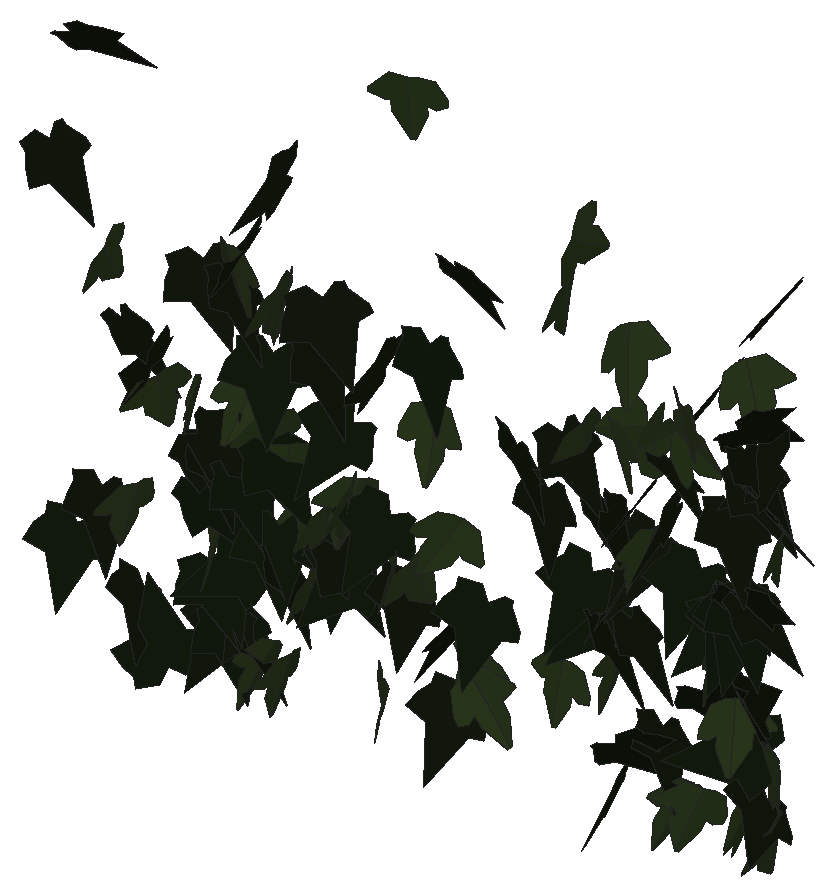
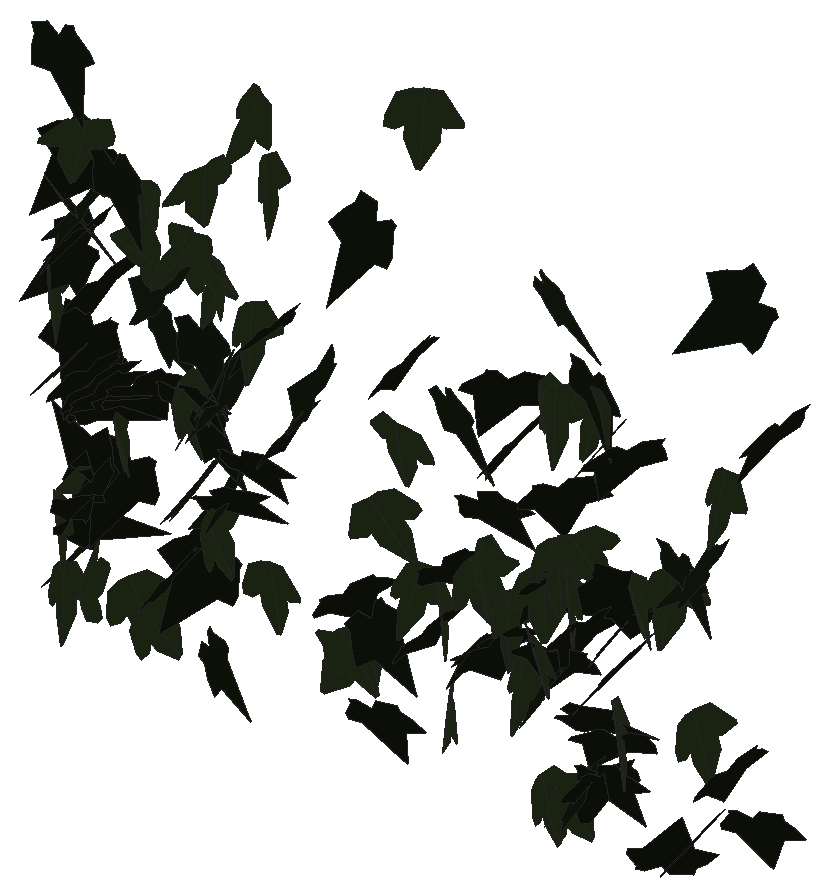
# SketchUp Ruby script. Lengths in inches.
U = 1.inch
M = Sketchup.active_model
def pt(a) = Geom::Point3d.new(a.map { |v| v * U })
def face(e, loops, mat)
  f = e.add_face(loops[0].map { |a| pt(a) })
  loops[1..].each { |l| e.add_face(l.map { |a| pt(a) }).erase! }
  f.material = f.back_material = mat if mat
  f
end
# faces: each face lists its corners as indices into pts; further lists are holes
def faces(e, pts, list, mat = nil) = list.each { |f| face(e, (f[0].is_a?(Array) ? f : [f]).map { |l| l.map { |i| pts[i] } }, mat) }
# xy, xz, yz: faces in a plane at the given z, y or x. An outline is a flat list of corners, or four numbers for a rectangle; further outlines are holes
def ring(l) = l.size == 4 ? [[l[0], l[1]], [l[2], l[1]], [l[2], l[3]], [l[0], l[3]]] : l.each_slice(2).to_a
def flat(e, list, mat, &to3) = list.each { |f| face(e, (f[0].is_a?(Array) ? f : [f]).map { |l| ring(l).map { |u, v| to3.(u, v) } }, mat) }
def xy(e, z, list, mat = nil) = flat(e, list, mat) { |x, y| [x, y, z] }
def xz(e, y, list, mat = nil) = flat(e, list, mat) { |x, z| [x, y, z] }
def yz(e, x, list, mat = nil) = flat(e, list, mat) { |y, z| [x, y, z] }
def lines(e, pts, list) = list.each { |a, b| e.add_line(pt(pts[a]), pt(pts[b])) }
# prism: a flat outline (further loops are holes) pulled along v
def prism(e, loops, v, mat = nil)
  f = face(e, loops, mat); d = Geom::Vector3d.new(v.map { |x| x * U })
  f.pushpull(f.normal.samedirection?(d) ? d.length : -d.length)
end
def box(e, o, s, mat = nil) = prism(e, [[o, [o[0] + s[0], o[1], o[2]], [o[0] + s[0], o[1] + s[1], o[2]], [o[0], o[1] + s[1], o[2]]]], [0, 0, s[2]], mat)
def at(x, y, z, deg = 0) = Geom::Transformation.translation(pt([x, y, z])) * Geom::Transformation.rotation(ORIGIN, Z_AXIS, deg.degrees)
def axes(o, x, y, z) = Geom::Transformation.new([*x, 0, *y, 0, *z, 0, *pt(o).to_a, 1])
def part(name) = M.definitions.add(name)
# library, detail: a bought-in or finely detailed component or shape, given as its bounding box
def library(name, o, s) = part(name).tap { |d| box(d.entities, o, s) }
def detail(e, o, s) = box(e.add_group.entities, o, s)
def put(e, d, t, mat = nil) = e.add_instance(d, t).tap { |i| i.material = mat if mat }
def group(e, t, mat = nil) = e.add_group.tap { |g| g.transformation = t; g.material = mat if mat }.entities
root = M.entities
M.materials.add("efeu1").color = [18, 25, 13]
M.materials.add("efeu2").color = [43, 57, 29]
c1 = part("ivyleaf_9")
p = [[1.54,2.16,1.25],[1.36,2.04,1.19],[-0.21,0.99,0.68],[-0.71,1.11,0.82],[-0.85,0.86,0.67],[-0.8,0.17,0.21],
  [-0.9,-0.01,0.1],[-0.67,-0.16,-0.02],[-0.08,-0.08,-0.05],[-0.03,-0.6,-0.4],[0.65,-0.88,-0.66],[0.83,-0.6,-0.49],
  [1.29,-0.42,-0.43],[1.8125,-0.07,-0.26],[1.21,0.44,0.15]]
faces(c1.entities,p,[[0,1,2,3,4,5,6,7,8,9,10,11,12,13,14]],"efeu1")
c2 = part("ivyleaf_10")
p = [[0,0.5,-0.03],[-0.0625,2.02,-0.43],[-0.19,2.01,-0.46],[-0.54,1.05,-0.29],[-0.52,0.625,-0.18],[-0.83,0.76,-0.28],
  [-1.16,0.64,-0.33],[-1.15,0.33,-0.24],[-0.77,-0.39,0.02],[-0.3,-0.51,0.16],[0.04,-0.48,0.23],[-0.02,2.01,-0.4375],
  [-0.06,2.01,-0.43],[0.04,-0.49,0.23],[0.67,-0.49,0.14],[1.38,0.36,-0.2],[1.375,0.51,-0.24],[0.81,0.65,-0.19],
  [0.62,0.59,-0.15],[0.6,1.09,-0.28],[0.5,1.23,-0.31]]
faces(c2.entities,p,[[0,1,2,3,4,5,6,7,8,9,10],[11,12,0,13,14,15,16,17,18,19,20]],"efeu2")
put(root,c1,axes([570.51,128.33,246.2],[0.79175,0.67685,0.12793],[0.09938,0.08063,-1.04162],[-0.68162,0.79795,-0.00327]))
put(root,c1,axes([574.61,129.34,255.92],[0.09837,-1.07427,-0.09221],[-0.0039,0.09224,-1.07876],[1.07822,0.09834,0.00451]))
put(root,c2,axes([560.36,128.3,244.3125],[0.17872,-0.33915,-0.98707],[-0.29964,0.94261,-0.37813],[0.99977,0.34313,0.06312]))
put(root,c2,axes([555.7,129.05,258.01],[0.38953,-1.0206,-0.04743],[0.00898,0.05417,-1.09206],[1.02167,0.38865,0.02768]))
put(root,c1,axes([558.13,129.76,247.77],[-0.63003,-0.67663,0.47075],[-0.08409,-0.53666,-0.88391],[0.81998,-0.57492,0.27105]))
put(root,c1,axes([575.53,128.6,253.44],[0.9103,0.44583,-0.40687],[-0.3516,-0.20676,-1.01321],[-0.4906,0.97542,-0.0288]))
put(root,c1,axes([553.1875,129.36,244.54],[-0.9432,-0.36605,-0.14838],[0.13024,0.07443,-1.0115],[0.37289,-0.95189,-0.02203]))
put(root,c2,axes([570.44,129,261.26],[0.29924,1.09198,-0.17073],[-0.0626,-0.15984,-1.1321],[-1.10348,0.30519,0.01793]))
put(root,c2,axes([567.76,128.87,262.32],[0.26589,-1.0177,-0.32096],[-0.01302,0.32766,-1.04972],[1.06704,0.2576,0.06717]))
put(root,c1,axes([552.43,128.7,251.47],[0.262,-0.23663,-1.0328],[0.64541,0.8794,-0.03776],[0.84031,-0.60165,0.35101]))
put(root,c2,axes([555.46,128.8125,257.78],[0.0348,-1.02892,-0.38326],[-0.01976,0.3828,-1.02949],[1.0978,0.03951,-0.00638]))
put(root,c1,axes([559.59,129.67,250.43],[-0.61367,-0.82906,0.1765],[-0.04965,-0.18236,-1.02925],[0.84619,-0.61195,0.0676]))
put(root,c1,axes([568.3125,129.49,251.38],[-0.92344,-0.44266,-0.19578],[0.22055,-0.00942,-1.01897],[0.43086,-0.94392,0.10198]))
put(root,c1,axes([554.17,128.48,258.89],[-0.38604,0.9338,0.36352],[-0.118,0.34449,-1.01023],[-0.99509,-0.40311,-0.02123]))
put(root,c1,axes([563.44,128.61,261.67],[1.03191,0.14353,-0.33162],[-0.33689,0.01922,-1.03998],[-0.13069,1.08372,0.06236]))
put(root,c1,axes([545.85,128.98,260.22],[0.38436,-0.88613,-0.4897],[-0.08753,0.49276,-0.96036],[1.00865,0.38044,0.10327]))
put(root,c1,axes([575.79,128.25,260.11],[0.64088,0.75897,0.40754],[0.23232,0.33686,-0.99267],[-0.82955,0.68069,0.03685]))
put(root,c1,axes([550.33,128.61,253.35],[-0.49106,0.85867,0.33268],[-0.1975,0.27005,-0.98853],[-0.89944,-0.5281,0.03543]))
put(root,c1,axes([576.62,129.05,258.65],[-0.95119,0.53547,0.04189],[-0.03882,0.01643,-1.09155],[-0.5357,-0.95197,0.00472]))
put(root,c1,axes([570.21,129.15,252.13],[-0.69709,0.647,-0.42557],[0.30379,-0.29823,-0.95102],[-0.71235,-0.76034,0.01088]))
put(root,c2,axes([573.12,129.34,244.56],[-0.65969,-0.67976,0.40464],[-0.1732,-0.38998,-0.9375],[0.77189,-0.66846,0.13546]))
put(root,c1,axes([572.12,129.31,255.32],[-0.81079,0.45568,-0.52869],[0.42804,-0.31545,-0.92833],[-0.5513,-0.91508,0.05675]))
put(root,c1,axes([555.57,129.18,262.24],[-0.89884,0.55758,-0.22216],[0.15773,-0.16655,-1.05619],[-0.57911,-0.91078,0.05714]))
put(root,c1,axes([570.72,128.79,255.07],[-0.43929,0.95911,-0.06774],[0.03807,-0.05707,-1.05487],[-0.96074,-0.4408,-0.01082]))
put(root,c2,axes([570.82,129.04,258.13],[-0.36458,0.14567,0.98024],[-0.98712,-0.14573,-0.34549],[0.08763,-1.03564,0.18649]))
put(root,c1,axes([555.17,129.42,248.53],[-0.50687,-0.74297,-0.51958],[0.48507,0.28066,-0.87454],[0.76595,-0.66941,0.21001]))
put(root,c2,axes([569.83,129.05,257.54],[-0.83895,0.59742,-0.21327],[0.13859,-0.17244,-1.02824],[-0.61902,-0.84829,0.05882]))
put(root,c1,axes([556.91,129.36,255.95],[0.3444,-1.00501,-0.12122],[0.00485,0.12968,-1.06137],[1.01229,0.3413,0.04633]))
put(root,c1,axes([575.24,129.26,258.5],[0.61903,-0.89247,-0.02327],[0.08023,0.08382,-1.08017],[0.88916,0.61377,0.11367]))
put(root,c1,axes([557.28,129.16,258.07],[-0.2616,-0.79135,-0.69858],[0.3032,0.63305,-0.83066],[1.0111,-0.39457,0.06835]))
put(root,c2,axes([549.05,129.27,247.82],[-0.19962,-1.01518,0.1203],[-0.0219,-0.1183,-1.03462],[1.02205,-0.20081,0.00132]))
put(root,c1,axes([567.5,129.17,256.51],[0.3953,-0.92591,-0.37005],[-0.02991,0.38688,-0.99997],[0.99667,0.37885,0.11677]))
put(root,c2,axes([562.8,129.15,251.25],[0.79173,0.45752,-0.55032],[-0.61351,0.01134,-0.87321],[-0.36849,0.96413,0.27142]))
put(root,c1,axes([574.6,129.77,252.11],[-0.2231,-1.0258,0.17771],[-0.01527,-0.1785,-1.04953],[1.04097,-0.22246,0.02269]))
put(root,c1,axes([575.49,129.9,245.05],[-0.12001,-0.90622,0.54631],[0.1383,-0.55853,-0.89611],[1.04908,-0.03004,0.18063]))
put(root,c1,axes([552.54,129.36,246.1875],[-0.20645,-0.83999,-0.54914],[0.46667,0.41598,-0.81175],[0.88846,-0.41368,0.29877]))
put(root,c2,axes([572.8,128.88,259.47],[-0.86177,0.59298,0.20748],[-0.1777,0.10774,-1.04601],[-0.60258,-0.87982,0.01175]))
put(root,c1,axes([575.44,129.04,253.1],[0.65623,-0.76037,-0.3642],[-0.05914,0.41887,-0.98107],[0.84102,0.62276,0.2152]))
put(root,c1,axes([554.8,129.5,254.95],[-0.44344,-0.91696,-0.33872],[0.14444,0.30639,-1.01855],[0.96679,-0.46636,-0.00318]))
put(root,c2,axes([550.4,128.98,252.625],[-0.44666,-0.93006,-0.29734],[0.09531,0.28389,-1.03114],[0.97177,-0.45533,-0.03554]))
put(root,c2,axes([573.62,129.48,250.59],[0.52614,-0.83541,0.33377],[0.25614,-0.23155,-0.98332],[0.86239,0.57846,0.08842]))
put(root,c1,axes([555.29,129.52,247.16],[0.48304,-0.90652,0.15769],[0.06767,-0.14261,-1.02716],[0.91765,0.48771,-0.00726]))
put(root,c1,axes([574.38,129.8125,251.87],[-0.33064,-0.97685,0.19643],[-0.09901,-0.17372,-1.03061],[0.99147,-0.34311,-0.03741]))
put(root,c2,axes([558.32,129.1,251.02],[0.27945,-1.01362,-0.26101],[-0.03217,0.2617,-1.05077],[1.04619,0.2788,0.03741]))
put(root,c2,axes([548.32,128.77,257.04],[-0.00325,-0.85845,-0.63854],[0.01889,0.63839,-0.85835],[1.06972,-0.01388,0.01322]))
put(root,c1,axes([565.125,129.71,255.02],[0.46523,-0.86766,0.51882],[0.23317,-0.46363,-0.98444],[0.98369,0.52025,-0.01202]))
put(root,c1,axes([552.13,128.96,249.35],[0.65301,-0.72226,-0.52996],[-0.14534,0.56171,-0.94461],[0.88396,0.62591,0.23619]))
put(root,c1,axes([558.01,129.65,253.41],[-0.97319,-0.41909,-0.03941],[0.03365,0.0215,-1.05957],[0.41959,-0.97375,-0.00643]))
put(root,c2,axes([574.68,129.22,248.41],[0.68235,0.80377,-0.07318],[-0.05299,-0.05101,-1.05432],[-0.80535,0.68437,0.00737]))
put(root,c1,axes([561.4,129.67,257.52],[0.14827,-1.05732,0.05783],[0.00175,-0.05815,-1.06765],[1.0589,0.14814,-0.00634]))
put(root,c2,axes([574.54,129.99,244.33],[0.0526,-0.06848,1.13998],[0.6386,-0.94434,-0.08619],[0.9468,0.64075,-0.00519]))
put(root,c1,axes([552.16,129.57,250.5],[0.37161,-0.96197,0.06849],[0.05308,-0.05289,-1.0308],[0.96294,0.37415,0.03039]))
put(root,c1,axes([553.94,129.72,246.68],[-0.92038,-0.13165,0.44521],[-0.40646,-0.24917,-0.91397],[0.22434,-0.99158,0.17056]))
put(root,c2,axes([553.45,129.17,258.4],[-0.93835,0.47195,-0.16449],[0.12226,-0.12253,-1.04897],[-0.48461,-0.94475,0.05388]))
put(root,c1,axes([553.11,129.42,244.43],[-0.0314,-0.92521,-0.4228],[-0.01906,0.42347,-0.92524],[1.01706,-0.02063,-0.0304]))
put(root,c2,axes([554.32,129.77,243.37],[0.01924,-0.88876,0.53137],[0.03745,-0.53052,-0.88869],[1.03482,0.03572,0.02228]))
put(root,c1,axes([559.81,129.14,256.37],[-0.74066,0.78649,0.00398],[-0.01204,-0.00588,-1.08027],[-0.78641,-0.74065,0.01279]))
put(root,c1,axes([555.02,129.26,251.61],[0.24268,-0.87891,-0.54607],[-0.01392,0.55806,-0.9044],[1.03464,0.21366,0.11591]))
put(root,c1,axes([568.99,129.5,249.68],[0.64507,-0.84105,0.05564],[0.0358,-0.04266,-1.05994],[0.84212,0.64606,0.00244]))
put(root,c2,axes([560.875,129.25,267.45],[-1.00586,-0.41148,0.06163],[-0.05208,-0.03545,-1.08669],[0.41279,-1.00712,0.01307]))
put(root,c2,axes([560.16,129.14,248.88],[0.44817,-0.86397,-0.43718],[-0.14609,0.41589,-0.97166],[0.9572,0.468,0.05639]))
put(root,c1,axes([571.5,129.76,256.73],[0.39036,-0.86605,0.48781],[0.41428,-0.33463,-0.92562],[0.90353,0.52759,0.21365]))
put(root,c1,axes([553.68,129.48,250.16],[0.11491,-0.97087,-0.37461],[0.00846,0.37775,-0.97641],[1.0406,0.10414,0.0493]))
put(root,c2,axes([570.53,129.77,253.21],[0.07899,-0.95431,0.43372],[0.18118,-0.41598,-0.94826],[1.03247,0.146,0.13322]))
put(root,c1,axes([550.61,129.17,241.95],[-0.9113,-0.43775,0.27809],[0.24587,0.13037,1.01093],[-0.45663,0.94382,-0.01066]))
put(root,c2,axes([572.03,129.875,244.12],[-0.14346,-0.8239,0.59513],[-0.01247,-0.59956,-0.83303],[1.01629,-0.12366,0.07379]))
put(root,c2,axes([554.91,129.37,252.4375],[-0.41636,-0.95888,-0.06122],[0.00986,0.06246,-1.04525],[0.96078,-0.41618,-0.01581]))
put(root,c1,axes([572.62,129.93,252.82],[-0.54296,-0.90726,0.00395],[-0.00182,-0.00351,-1.05732],[0.90727,-0.54297,0.00024]))
put(root,c1,axes([552.98,129.63,257.16],[0.44408,-0.96053,-0.05264],[0.01317,0.06405,-1.0575],[0.96188,0.44257,0.03879]))
put(root,c2,axes([555.29,129.58,243.33],[0.05771,-1.0048,0.10155],[-0.00334,-0.10191,-1.00641],[1.00991,0.05709,-0.00913]))
put(root,c1,axes([546.26,129.74,245.38],[-0.72995,-0.59799,-0.36276],[0.28516,0.22434,-0.9436],[0.63866,-0.78364,0.00669]))
put(root,c1,axes([574.55,129.7,248.6],[-0.05519,-0.06408,1.06097],[0.73609,-0.76871,-0.00814],[0.76676,0.73335,0.08418]))
put(root,c1,axes([560.21,130.05,247.75],[-0.09151,-1.02117,0.24086],[0.02689,-0.24398,-1.02417],[1.04885,-0.08284,0.04727]))
put(root,c1,axes([573.7,128.93,249.05],[0.81459,0.65168,-0.14431],[-0.10598,-0.09852,-1.04313],[-0.659,0.82138,-0.01063]))
put(root,c1,axes([575.27,129.44,257.69],[0.44235,-0.90867,-0.3788],[0.00013,0.41533,-0.99616],[0.98446,0.40823,0.17033]))
put(root,c1,axes([568.76,129.08,254.38],[0.90877,-0.34909,-0.4459],[-0.33567,0.34699,-0.95576],[0.45609,0.95094,0.18506]))
put(root,c1,axes([574.02,130.16,251.6],[-0.75057,-0.65112,0.33645],[-0.13687,-0.34857,-0.97993],[0.72001,-0.74502,0.16444]))
put(root,c1,axes([574.33,130.06,248.25],[0.25448,-0.52196,1.01173],[0.50317,-0.87837,-0.57972],[1.0212,0.56287,0.03353]))
put(root,c2,axes([571.53,128.62,257.77],[0.00062,0.13162,1.05151],[-0.34693,0.99359,-0.12416],[-1.00132,-0.34418,0.04367]))
put(root,c1,axes([575.36,129.23,256.93],[1.05649,-0.2578,-0.00147],[0.00224,0.01542,-1.08738],[0.25779,1.05638,0.01551]))
put(root,c1,axes([570.69,129.875,253.26],[-0.97575,-0.34148,-0.20869],[0.21804,0.00754,-1.03181],[0.33558,-0.99779,0.06362]))
put(root,c1,axes([551.84,129.6,257.46],[-0.04314,-0.93139,-0.50119],[0.16111,0.48997,-0.9244],[1.04534,-0.11395,0.12179]))
put(root,c2,axes([568.34,128.79,264.51],[-0.01096,-0.65902,-0.96601],[0.11998,0.96032,-0.6565],[1.16322,-0.10526,0.05862]))
put(root,c2,axes([572.1,129.67,257.78],[0.06481,0.0127,1.18772],[1.18215,-0.11645,-0.06326],[0.11559,1.18378,-0.01897]))
put(root,c2,axes([567.16,129.55,247.27],[-1.02559,0.1001,0.18014],[-0.20146,-0.29426,-0.98343],[-0.04343,-0.99885,0.30777]))
put(root,c2,axes([555.7,129.66,248.77],[0.86434,-0.57614,0.0617],[0.05486,-0.02894,-1.03874],[0.57683,0.86606,0.00634]))
put(root,c1,axes([574.78,129.79,252.54],[-0.02355,-1.03029,-0.27005],[-0.00166,0.27015,-1.03053],[1.06509,-0.02236,-0.00758]))
put(root,c2,axes([561.49,129.64,254.81],[1.10941,-0.10197,0.14703],[0.14623,-0.01543,-1.11409],[0.10312,1.11901,-0.00197]))
put(root,c2,axes([561.0625,129.19,249.2],[-0.23849,-0.87585,-0.50942],[0.17494,0.47989,-0.90698],[0.99801,-0.29342,0.03725]))
put(root,c2,axes([563.61,129.38,245.4],[0.80424,0.2367,0.68994],[0.63759,0.2707,-0.83609],[-0.35429,1.02447,0.06152]))
put(root,c1,axes([548.77,130.18,243.65],[0.03211,-0.95359,0.40649],[0.08293,-0.40302,-0.95199],[1.03329,0.06198,0.06377]))
put(root,c2,axes([568.04,129.35,256.79],[-0.05058,-1.0225,-0.34592],[0.02084,0.34531,-1.02375],[1.07923,-0.05459,0.00356]))
put(root,c1,axes([575.3,129.99,246.77],[-0.7712,-0.11484,0.84238],[-0.8292,-0.14946,-0.77951],[0.18767,-1.13226,0.01746]))
put(root,c2,axes([558.06,129.86,250.81],[-0.35476,-0.93148,0.34824],[0.02319,-0.37739,-0.98581],[0.99417,-0.32358,0.14726]))
put(root,c2,axes([575.23,129.36,261.47],[0.57305,0.89184,0.18458],[0.08497,0.16478,-1.05994],[-0.90677,0.57905,0.01733]))
put(root,c2,axes([553.78,129.75,253.32],[0.71054,0.66056,-0.44439],[-0.33633,-0.29082,-0.97006],[-0.7216,0.78599,0.01455]))
put(root,c1,axes([547.22,129.95,247.03],[0.03403,-1.0252,-0.03651],[-0.00624,0.03632,-1.02575],[1.02583,0.03423,-0.00502]))
put(root,c2,axes([556.61,129.16,247.11],[0.0495,-0.82381,-0.61806],[-0.03775,0.6169,-0.82529],[1.02919,0.06225,-0.00054]))
put(root,c2,axes([551.22,129.84,252.18],[0.58536,-0.83707,0.25306],[0.15669,-0.1992,-1.02134],[0.86033,0.60581,0.01383]))
put(root,c2,axes([557,129.48,249.66],[0.04386,-1.04284,-0.2309],[0.00094,0.23114,-1.04371],[1.0681,0.04262,0.0104]))
put(root,c2,axes([569.28,129.92,248.5],[0.21258,-0.97969,0.34164],[0.08677,-0.33073,-1.00239],[1.03392,0.22919,0.01388]))
put(root,c1,axes([563.42,130.14,248.21],[-0.40201,-0.96985,0.04167],[0.01704,-0.05214,-1.04926],[0.9706,-0.40078,0.03568]))
put(root,c2,axes([552.34,129.43,247.01],[0.58831,-0.94171,-0.38932],[-0.12178,0.38135,-1.10646],[1.01171,0.59351,0.0932]))
put(root,c1,axes([576.41,129.21,264.5],[-0.34974,1.02892,-0.0112],[-0.02511,-0.02036,-1.08631],[-1.02867,-0.34933,0.03033]))
put(root,c1,axes([548.48,129.57,254.06],[0.75128,-0.75957,-0.11396],[0.05409,0.21134,-1.05203],[0.76617,0.72989,0.18602]))
put(root,c1,axes([566.01,130.14,253.44],[0.15955,-1.01846,0.19997],[-0.00609,-0.20323,-1.03023],[1.03789,0.15537,-0.03678]))
put(root,c1,axes([568.84,130.22,250.04],[-0.92759,-0.435,0.22936],[-0.13692,-0.24184,-1.01243],[0.47231,-0.92441,0.15694]))
put(root,c1,axes([546.82,129.05,264.68],[1.01504,0.24664,0.30481],[0.26254,0.20077,-1.03673],[-0.29123,1.04063,0.12778]))
put(root,c2,axes([555.33,129.66,251.3],[-0.71189,-0.77935,0.03393],[0.0328,-0.07579,-1.05286],[0.7794,-0.70866,0.07529]))
put(root,c1,axes([569.44,129.22,254.18],[0.70825,-0.38353,-0.67717],[-0.49375,0.48628,-0.79184],[0.60155,0.85071,0.14734]))
put(root,c2,axes([576.41,129.56,255.52],[0.3962,-0.96529,-0.257],[-0.00665,0.27392,-1.0391],[0.99889,0.38469,0.09501]))
put(root,c1,axes([573.96,129.3,260.48],[-0.45951,0.96714,0.04112],[-0.02115,0.03548,-1.07075],[-0.96778,-0.45998,0.00387]))
put(root,c1,axes([571.01,130.07,246.17],[0.22936,-1.0033,0.0634],[-0.00068,-0.06518,-1.02908],[1.00531,0.22886,-0.01516]))
put(root,c1,axes([557.65,129.66,248.39],[0.4145,-0.89348,-0.41572],[-0.04045,0.43519,-0.97566],[0.98463,0.39401,0.13492]))
put(root,c1,axes([569.4,129.83,243.8],[-0.70037,0.55446,-0.49499],[0.39506,-0.29839,-0.89322],[-0.62957,-0.80405,-0.00985]))
put(root,c2,axes([554.23,129.63,251.54],[0.76963,-0.73395,-0.13089],[0.05368,0.24219,-1.0424],[0.74359,0.74217,0.21072]))
put(root,c2,axes([576.2,129.46,246.72],[0.74542,-0.61204,-0.39838],[-0.12557,0.45337,-0.93147],[0.7194,0.71331,0.25021]))
put(root,c1,axes([569.94,129.79,250],[0.56681,-0.86114,-0.13041],[-0.01584,0.14537,-1.02881],[0.87081,0.56316,0.06617]))
put(root,c2,axes([575.96,129.48,244.11],[0.05587,-0.99685,-0.41769],[-0.04803,0.41555,-0.99815],[1.07975,0.07007,-0.02279]))
put(root,c2,axes([570.28,129.9,253.08],[0.07503,-1.03808,0.12585],[0.03161,-0.12387,-1.04054],[1.0452,0.07826,0.02243]))
put(root,c1,axes([557.21,130.1875,248.36],[-0.20094,-1.02571,-0.0328],[-0.01368,0.0361,-1.04501],[1.02615,-0.20038,-0.02036]))
put(root,c2,axes([563.69,129.84,246.06],[-0.79971,0.00914,0.62017],[-0.58705,-0.33774,-0.75202],[0.20018,-0.95398,0.27218]))
put(root,c1,axes([562.51,129.79,247.32],[-0.40673,0.78081,-0.50896],[0.11563,-0.50875,-0.87289],[-0.92484,-0.40699,0.1147]))
put(root,c1,axes([553.4,129.87,244.07],[0.67045,-0.77657,-0.01064],[-0.00207,0.01227,-1.02593],[0.77664,0.67043,0.00645]))
put(root,c1,axes([562.24,130.11,244.14],[-0.89269,-0.44177,-0.30747],[0.27219,0.14318,-0.996],[0.46434,-0.93324,-0.00727]))
